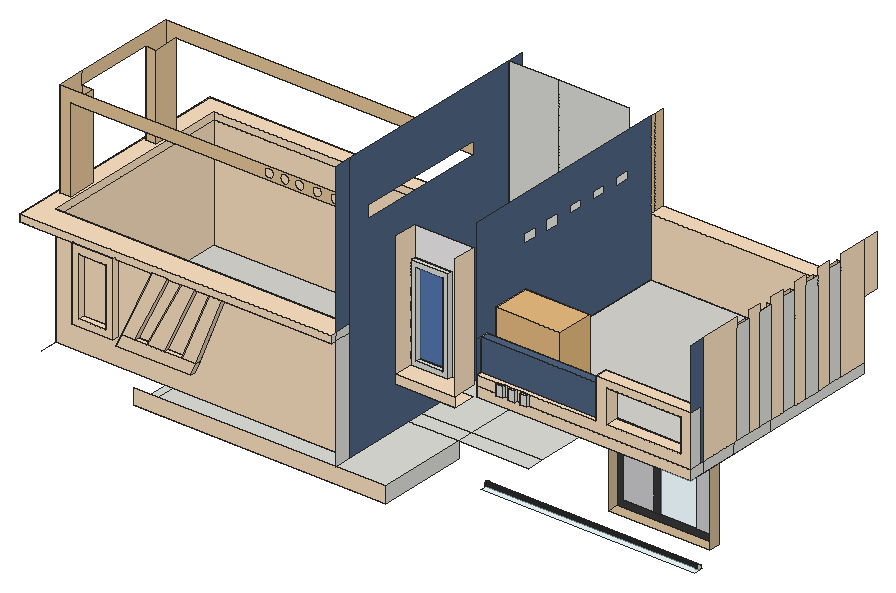
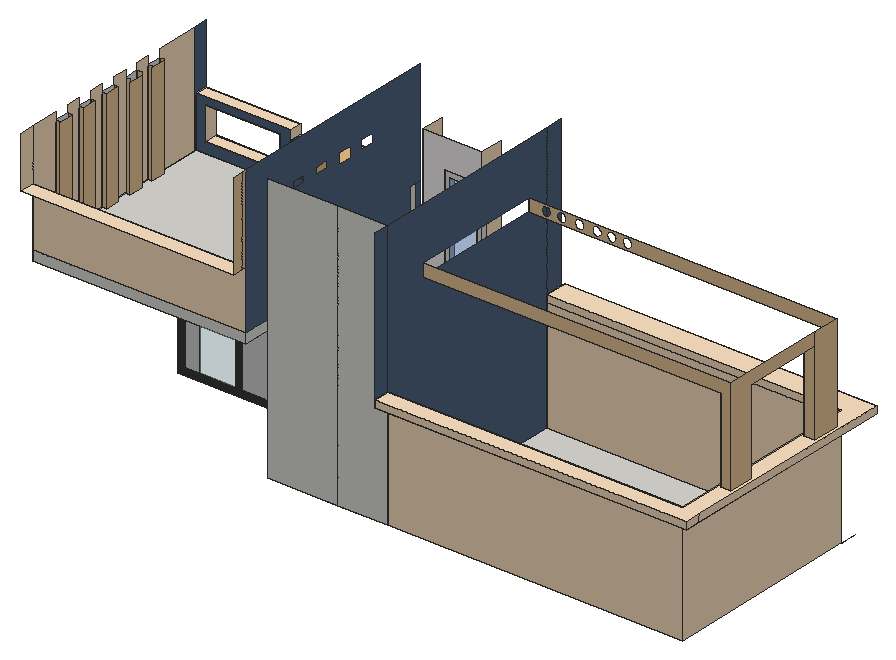
# SketchUp Ruby script. Lengths in inches.
U = 1.inch
M = Sketchup.active_model
def pt(a) = Geom::Point3d.new(a.map { |v| v * U })
def face(e, loops, mat)
  f = e.add_face(loops[0].map { |a| pt(a) })
  loops[1..].each { |l| e.add_face(l.map { |a| pt(a) }).erase! }
  f.material = f.back_material = mat if mat
  f
end
# faces: each face lists its corners as indices into pts; further lists are holes
def faces(e, pts, list, mat = nil) = list.each { |f| face(e, (f[0].is_a?(Array) ? f : [f]).map { |l| l.map { |i| pts[i] } }, mat) }
# xy, xz, yz: faces in a plane at the given z, y or x. An outline is a flat list of corners, or four numbers for a rectangle; further outlines are holes
def ring(l) = l.size == 4 ? [[l[0], l[1]], [l[2], l[1]], [l[2], l[3]], [l[0], l[3]]] : l.each_slice(2).to_a
def flat(e, list, mat, &to3) = list.each { |f| face(e, (f[0].is_a?(Array) ? f : [f]).map { |l| ring(l).map { |u, v| to3.(u, v) } }, mat) }
def xy(e, z, list, mat = nil) = flat(e, list, mat) { |x, y| [x, y, z] }
def xz(e, y, list, mat = nil) = flat(e, list, mat) { |x, z| [x, y, z] }
def yz(e, x, list, mat = nil) = flat(e, list, mat) { |y, z| [x, y, z] }
def lines(e, pts, list) = list.each { |a, b| e.add_line(pt(pts[a]), pt(pts[b])) }
# prism: a flat outline (further loops are holes) pulled along v
def prism(e, loops, v, mat = nil)
  f = face(e, loops, mat); d = Geom::Vector3d.new(v.map { |x| x * U })
  f.pushpull(f.normal.samedirection?(d) ? d.length : -d.length)
end
def box(e, o, s, mat = nil) = prism(e, [[o, [o[0] + s[0], o[1], o[2]], [o[0] + s[0], o[1] + s[1], o[2]], [o[0], o[1] + s[1], o[2]]]], [0, 0, s[2]], mat)
def at(x, y, z, deg = 0) = Geom::Transformation.translation(pt([x, y, z])) * Geom::Transformation.rotation(ORIGIN, Z_AXIS, deg.degrees)
def axes(o, x, y, z) = Geom::Transformation.new([*x, 0, *y, 0, *z, 0, *pt(o).to_a, 1])
def part(name) = M.definitions.add(name)
# library, detail: a bought-in or finely detailed component or shape, given as its bounding box
def library(name, o, s) = part(name).tap { |d| box(d.entities, o, s) }
def detail(e, o, s) = box(e.add_group.entities, o, s)
def put(e, d, t, mat = nil) = e.add_instance(d, t).tap { |i| i.material = mat if mat }
def group(e, t, mat = nil) = e.add_group.tap { |g| g.transformation = t; g.material = mat if mat }.entities
root = M.entities
M.materials.add("[0012_Bisque]").color = [255, 228, 196]
M.materials.add("[0035_Tan]").color = [234, 201, 156]
M.materials.add("[Blinds Vertical Pattern]1").color = [212, 212, 214]
M.materials.add("[Color M07]").color = [58, 58, 58]
M.materials.add("[Formica Beige]").color = [211, 187, 149]
M.materials.add("[Formica Graystone]").color = [149, 146, 135]
M.materials.add("[Leather Blue]").color = [80, 102, 132]
M.materials.add("[Stone Vein Gray]1").color = [247, 245, 245]
M.materials.add("[Terrazzo Tile Light]").color = [219, 217, 210]
M.materials.add("[Translucent Glass Blue]").color = [100, 149, 237]
M.materials["[Translucent Glass Blue]"].alpha = 0.5
M.materials.add("[Translucent Glass Safety]").color = [204, 235, 244]
M.materials["[Translucent Glass Safety]"].alpha = 0.5
c1 = library("Flora+17",[-57.52,158.6,-38.64],[66.99,62.88,77.28])
xy(root,862.4375,[[187.18,439.49,197.99,595.47],[197.99,439.49,607.9,595.47],[607.9,439.49,615.34,595.47],[138.99,595.47,228.43,623.86]])
xy(root,863.95,[[860.01,607.94,1033.1875,626.38]],"[Formica Beige]")
xy(root,889,[[529.97,439.49,615.34,595.47],[529.97,595.47,615.34,623.86],[615.34,595.47,733.59,623.86],[529.97,623.86,615.34,808.22],[615.34,623.86,733.59,808.22]])
xy(root,889,[[28.68,470.4375,529.97,808.22]],"[Terrazzo Tile Light]")
xy(root,933.85,[[771.27,448.03,1134.07,465.29]],"[Translucent Glass Safety]")
xy(root,947.54,[[162.87,431.49,290.72,439.49]],"[0012_Bisque]")
xy(root,956.62,[[89.49,428.49,159.99,439.49]],"[0012_Bisque]")
xy(root,967.96,[[172.3,431.49,195.38,439.49],[215.64,431.49,245.26,439.49],[274.875,431.49,298.76,439.49]])
xy(root,967.96,[[195.38,431.49,215.64,439.49],[245.26,431.49,274.875,439.49]],"[0012_Bisque]")
xy(root,968.65,[[101.71,428.49,147.77,439.49]],"[0012_Bisque]")
xy(root,1037.12,[[860.01,607.94,1033.1875,626.38]],"[Formica Beige]")
xy(root,1050.61,[[633.21,439.49,733.59,477.49]],"[0012_Bisque]")
xy(root,1067.2,[[633.21,470.42,696.47,478.61]])
xy(root,1067.2,[[633.21,439.49,733.59,439.49,733.59,478.61,696.47,478.61,696.47,470.42,633.21,470.42]],"[0012_Bisque]")
xy(root,1067.59,[[101.71,428.49,147.77,439.49]])
xy(root,1075.63,[[641.64,470.42,688.04,478.61]])
xy(root,1079.8125,[[89.49,428.49,159.99,431.49],[0,431.49,89.49,439.49],[89.49,431.49,159.99,439.49],[159.99,431.49,223.93,439.49],[223.93,431.49,250.55,439.49],
  [250.55,431.49,273.98,439.49],[273.98,431.49,297.72,439.49],[297.72,431.49,321.46,439.49],[321.46,431.49,342.79,439.49],[342.79,431.49,529.97,439.49],
  [0,439.49,0,835.03,529.97,835.03,529.97,808.22,28.68,808.22,28.68,470.4375,529.97,470.4375,529.97,439.49],[771.27,607.94,1134.07,808.22]])
xy(root,1079.8125,[[771.27,439.49,1134.07,607.94]],"[Leather Blue]")
xy(root,1092.125,[[[0,431.49,529.97,431.49,529.97,470.4375,28.68,470.4375,28.68,808.22,529.97,808.22,529.97,835.03,0,835.03],[5.5,509.25,23.8,555.46],[5.5,690.86,23.8,733.33]]],"[0012_Bisque]")
xy(root,1096.75,[[807.07,434.86,817.84,439.49],[827.75,434.86,838.53,439.49],[848.07,434.86,858.84,439.49],[771.27,439.49,1134.07,460.91],[1126.57,539.27,1134.07,560.75],
  [1126.57,560.75,1134.07,563.87],[1126.57,586.45,1134.07,607.94],[1126.57,607.94,1134.07,611.06],[1126.57,636.14,1134.07,660.75],[1126.57,685.02,1134.07,709.62],
  [1126.57,734.95,1134.07,759.56]])
xy(root,1096.75,[[771.27,460.91,1134.07,460.91,1134.07,539.27,1126.57,539.27,1126.57,563.87,1134.07,563.87,1134.07,586.45,1126.57,586.45,1126.57,611.06,1134.07,611.06,1134.07,636.14,1126.57,636.14,1126.57,660.75,1134.07,660.75,1134.07,685.02,1126.57,685.02,1126.57,709.62,1134.07,709.62,1134.07,734.95,1126.57,734.95,1126.57,759.56,1134.07,759.56,1134.07,808.22,771.27,808.22]],"[Terrazzo Tile Light]")
xy(root,1114.1875,[[807.07,434.86,817.84,439.49],[827.75,434.86,838.53,439.49],[848.07,434.86,858.84,439.49],[771.27,447.3,973.24,460.91]])
xy(root,1114.1875,[[771.27,439.49,973.24,447.3]],"[0012_Bisque]")
xy(root,1115.04,[[991.23,439.49,1117.66,460.91]],"[0012_Bisque]")
xy(root,1167.875,[[771.27,447.3,973.24,460.91]],"[Leather Blue]")
xy(root,1171.5,[[991.23,439.49,1117.66,460.91]])
xy(root,1182.875,[[973.24,439.49,1134.07,460.91]],"[0012_Bisque]")
xy(root,1197.6875,[[771.27,808.22,1134.07,835.03]],"[0012_Bisque]")
xy(root,1218.53,[[641.64,470.42,688.04,478.61]])
xy(root,1226.96,[[633.21,470.42,696.47,478.61]])
xz(root,428.49,[[[89.49,956.62,159.99,1079.8125],[101.71,968.65,147.77,1067.59]]],"[0012_Bisque]")
xz(root,431.49,[[162.87,947.54,290.72,947.54,298.76,967.96,172.3,967.96],[172.3,967.96,195.38,967.96,250.55,1079.8125,223.93,1079.8125],[215.64,967.96,245.26,967.96,297.72,1079.8125,273.98,1079.8125],[274.875,967.96,298.76,967.96,342.79,1079.8125,321.46,1079.8125],[0,1079.8125,529.97,1092.125]],"[0012_Bisque]")
xz(root,434.86,[[807.07,1096.75,817.84,1114.1875],[827.75,1096.75,838.53,1114.1875],[848.07,1096.75,858.84,1114.1875]])
xz(root,439.49,[[162.87,947.54,172.3,967.96,298.76,967.96,290.72,947.54],[[89.49,956.62,159.99,1079.8125],[101.71,968.65,147.77,1067.59]],[172.3,967.96,223.93,1079.8125,250.55,1079.8125,195.38,967.96],[215.64,967.96,273.98,1079.8125,297.72,1079.8125,245.26,967.96],[274.875,967.96,321.46,1079.8125,342.79,1079.8125,298.76,967.96],
  [807.07,1096.75,817.84,1114.1875],[827.75,1096.75,838.53,1114.1875],[848.07,1096.75,858.84,1114.1875]])
xz(root,439.49,[[187.18,862.4375,615.34,889],[195.38,967.96,215.64,967.96,273.98,1079.8125,250.55,1079.8125],[245.26,967.96,274.875,967.96,321.46,1079.8125,297.72,1079.8125],[101.71,968.65,147.77,1067.59],[633.21,1050.61,733.59,1067.2],
  [771.27,1079.8125,1134.07,1096.75],[771.27,1096.75,807.07,1114.1875],[817.84,1096.75,827.75,1114.1875],[838.53,1096.75,848.07,1114.1875],[[858.84,1096.75,1134.07,1096.75,1134.07,1182.875,973.24,1182.875,973.24,1114.1875,858.84,1114.1875],[991.23,1115.04,1117.66,1171.5]]],"[0012_Bisque]")
xz(root,447.3,[[771.27,1114.1875,973.24,1167.875]],"[Leather Blue]")
xz(root,460.91,[[[771.27,1096.75,771.27,1114.1875,973.24,1114.1875,973.24,1182.875,1134.07,1182.875,1134.07,1096.75],[991.23,1115.04,1117.66,1171.5]],[771.27,1114.1875,973.24,1167.875]],"[Leather Blue]")
xz(root,470.42,[[[633.21,1067.2,696.47,1226.96],[641.64,1075.63,688.04,1218.53]]])
xz(root,470.4375,[[28.68,889,529.97,1079.8125],[28.68,1079.8125,529.97,1092.125]],"[0012_Bisque]")
xz(root,478.61,[[[633.21,1067.2,696.47,1226.96],[641.64,1075.63,688.04,1218.53]]])
xz(root,478.61,[[696.47,1067.2,733.59,1067.2,733.59,1276.62,633.21,1276.62,633.21,1226.96,696.47,1226.96]],"[Stone Vein Gray]1")
xz(root,478.61,[[641.64,1075.63,688.04,1218.53]],"[Translucent Glass Blue]")
xz(root,509.25,[[[5.5,1092.125,23.8,1092.125,23.8,1235.23,529.97,1235.23,529.97,1256.625,5.5,1256.625],[473.26,1238.66,471.24,1238.93,469.35,1239.71,467.74,1240.95,466.49,1242.57,465.71,1244.45,465.45,1246.48,465.71,1248.5,466.49,1250.38,467.74,1252,469.35,1253.24,471.24,1254.02,473.26,1254.29,475.28,1254.02,477.17,1253.24,478.78,1252,480.03,1250.38,480.81,1248.5,481.07,1246.48,480.81,1244.45,480.03,1242.57,478.78,1240.95,477.17,1239.71,475.28,1238.93],[413.2,1238.66,411.18,1238.93,409.29,1239.71,407.67,1240.95,406.43,1242.57,405.65,1244.45,405.38,1246.48,405.65,1248.5,406.43,1250.38,407.67,1252,409.29,1253.24,411.18,1254.02,413.2,1254.29,415.22,1254.02,417.1,1253.24,418.72,1252,419.96,1250.38,420.74,1248.5,421.01,1246.48,420.74,1244.45,419.96,1242.57,418.72,1240.95,417.1,1239.71,415.22,1238.93],[442.88,1238.66,440.86,1238.93,438.98,1239.71,437.36,1240.95,436.12,1242.57,435.34,1244.45,435.07,1246.48,435.34,1248.5,436.12,1250.38,437.36,1252,438.98,1253.24,440.86,1254.02,442.88,1254.29,444.91,1254.02,446.79,1253.24,448.41,1252,449.65,1250.38,450.43,1248.5,450.7,1246.48,450.43,1244.45,449.65,1242.57,448.41,1240.95,446.79,1239.71,444.91,1238.93],[388.01,1238.66,385.99,1238.93,384.1,1239.71,382.49,1240.95,381.24,1242.57,380.46,1244.45,380.2,1246.48,380.46,1248.5,381.24,1250.38,382.49,1252,384.1,1253.24,385.99,1254.02,388.01,1254.29,390.03,1254.02,391.92,1253.24,393.53,1252,394.78,1250.38,395.56,1248.5,395.82,1246.48,395.56,1244.45,394.78,1242.57,393.53,1240.95,391.92,1239.71,390.03,1238.93],[499.45,1238.66,497.43,1238.93,495.54,1239.71,493.92,1240.95,492.68,1242.57,491.9,1244.45,491.63,1246.48,491.9,1248.5,492.68,1250.38,493.92,1252,495.54,1253.24,497.43,1254.02,499.45,1254.29,501.47,1254.02,503.35,1253.24,504.97,1252,506.21,1250.38,506.99,1248.5,507.26,1246.48,506.99,1244.45,506.21,1242.57,504.97,1240.95,503.35,1239.71,501.47,1238.93],[361.45,1238.66,359.43,1238.93,357.54,1239.71,355.92,1240.95,354.68,1242.57,353.9,1244.45,353.63,1246.48,353.9,1248.5,354.68,1250.38,355.92,1252,357.54,1253.24,359.43,1254.02,361.45,1254.29,363.47,1254.02,365.35,1253.24,366.97,1252,368.21,1250.38,368.99,1248.5,369.26,1246.48,368.99,1244.45,368.21,1242.57,366.97,1240.95,365.35,1239.71,363.47,1238.93]]],"[0035_Tan]")
xz(root,539.27,[[1126.57,1096.75,1134.07,1271.79]],"[0035_Tan]")
xz(root,555.46,[[5.5,1092.125,23.8,1235.23]],"[0035_Tan]")
xz(root,563.87,[[1126.57,1096.75,1134.07,1271.79]],"[0035_Tan]")
xz(root,586.45,[[1126.57,1096.75,1134.07,1272.79]],"[0035_Tan]")
xz(root,611.06,[[1126.57,1096.75,1134.07,1272.79]],"[0035_Tan]")
xz(root,626.38,[[871.74,875.67,922.51,1025.4],[996.07,875.67,1021.47,1025.4]],"[Blinds Vertical Pattern]1")
xz(root,626.38,[[[860.01,863.95,1033.1875,1037.12],[871.74,875.67,1021.47,1025.4]],[922.51,875.67,933.66,1025.4]],"[Color M07]")
xz(root,626.38,[[933.66,875.67,996.07,1025.4]],"[Translucent Glass Safety]")
xz(root,636.14,[[1126.57,1096.75,1134.07,1272.79]],"[0035_Tan]")
xz(root,660.75,[[1126.57,1096.75,1134.07,1272.79]],"[0035_Tan]")
xz(root,685.02,[[1126.57,1096.75,1134.07,1272.79]],"[0035_Tan]")
xz(root,690.86,[[5.5,1092.125,23.8,1235.23]],"[0035_Tan]")
xz(root,709.62,[[1126.57,1096.75,1134.07,1272.79]],"[0035_Tan]")
xz(root,733.33,[[5.5,1092.125,5.5,1256.625,529.97,1256.625,529.97,1235.23,23.8,1235.23,23.8,1092.125]],"[0035_Tan]")
xz(root,734.95,[[1126.57,1096.75,1134.07,1272.79]],"[0035_Tan]")
xz(root,759.56,[[1126.57,1096.75,1134.07,1272.79]],"[0035_Tan]")
xz(root,808.22,[[529.97,889,615.34,1345.9375],[615.34,889,733.59,1345.9375],[771.27,1079.8125,1134.07,1096.75]])
xz(root,808.22,[[28.68,889,529.97,1079.8125],[28.68,1079.8125,529.97,1092.125],[771.27,1096.75,1134.07,1197.6875]],"[0012_Bisque]")
xz(root,835.03,[[0,1079.8125,529.97,1092.125]],"[0012_Bisque]")
yz(root,0,[[431.49,1079.8125,808.22,1092.125],[808.22,1079.8125,835.03,1092.125]],"[0012_Bisque]")
yz(root,5.5,[[509.25,1092.125,555.46,1256.625],[690.86,1092.125,690.86,1235.23,555.46,1235.23,555.46,1256.625,733.33,1256.625,733.33,1092.125]],"[0035_Tan]")
yz(root,23.8,[[509.25,1092.125,555.46,1235.23],[690.86,1092.125,733.33,1235.23]],"[0035_Tan]")
yz(root,28.68,[[470.4375,889,808.22,1079.8125],[470.4375,1079.8125,808.22,1092.125]],"[0012_Bisque]")
yz(root,89.49,[[428.49,956.62,439.49,1079.8125]],"[0012_Bisque]")
yz(root,101.71,[[428.49,968.65,439.49,1067.59]],"[0012_Bisque]")
yz(root,147.77,[[428.49,968.65,439.49,1067.59]],"[0012_Bisque]")
yz(root,159.99,[[428.49,956.62,439.49,1079.8125]],"[0012_Bisque]")
yz(root,529.97,[[439.49,889,470.4375,1079.8125],[431.49,1079.8125,439.49,1092.125],[439.49,1079.8125,470.4375,1092.125],[808.22,1079.8125,835.03,1092.125]])
yz(root,529.97,[[[470.4375,889,808.22,1345.9375],[509.25,1235.23,733.33,1256.625]],[439.49,1092.125,470.4375,1345.9375],[808.22,1092.125,835.03,1345.9375]],"[Leather Blue]")
yz(root,615.34,[[439.49,862.4375,595.47,889]])
yz(root,633.21,[[470.42,1067.2,478.61,1226.96]])
yz(root,633.21,[[439.49,1067.2,470.42,1067.2,470.42,1226.96,478.61,1226.96,478.61,1276.62,439.49,1276.62]],"[0012_Bisque]")
yz(root,641.64,[[470.42,1075.63,478.61,1218.53]])
yz(root,688.04,[[470.42,1075.63,478.61,1218.53]])
yz(root,696.47,[[470.42,1067.2,478.61,1226.96]])
yz(root,733.59,[[439.49,1067.2,478.61,1276.62]],"[0012_Bisque]")
yz(root,771.27,[[439.49,1079.8125,808.22,1096.75],[439.49,1096.75,460.91,1114.1875],[447.3,1114.1875,460.91,1167.875]])
yz(root,771.27,[[808.22,1197.6875,817.66,1345.9375],[817.66,1197.6875,835.03,1345.9375]],"[0035_Tan]")
yz(root,771.27,[[[460.91,1096.75,808.22,1096.75,808.22,1345.9375,439.49,1345.9375,439.49,1167.875,460.91,1167.875],[586.45,1266.48,611.06,1284.8125],[539.27,1268.97,563.87,1284.8125],[734.95,1271.04,759.56,1284.8125],[636.14,1272.79,660.75,1284.8125],[685.02,1272.79,709.62,1284.8125]],[439.49,1114.1875,447.3,1167.875]],"[Leather Blue]")
yz(root,807.07,[[434.86,1096.75,439.49,1114.1875]])
yz(root,817.84,[[434.86,1096.75,439.49,1114.1875]])
yz(root,827.75,[[434.86,1096.75,439.49,1114.1875]])
yz(root,838.53,[[434.86,1096.75,439.49,1114.1875]])
yz(root,848.07,[[434.86,1096.75,439.49,1114.1875]])
yz(root,858.84,[[434.86,1096.75,439.49,1114.1875]])
yz(root,860.01,[[607.94,863.95,626.38,1037.12]],"[Formica Beige]")
yz(root,973.24,[[447.3,1114.1875,460.91,1167.875]])
yz(root,973.24,[[439.49,1114.1875,447.3,1167.875],[439.49,1167.875,460.91,1182.875]],"[0012_Bisque]")
yz(root,991.23,[[439.49,1115.04,460.91,1171.5]],"[0012_Bisque]")
yz(root,1033.1875,[[607.94,863.95,626.38,1037.12]],"[Formica Beige]")
yz(root,1117.66,[[439.49,1115.04,460.91,1171.5]],"[0012_Bisque]")
yz(root,1126.57,[[539.27,1096.75,563.87,1268.97],[586.45,1096.75,611.06,1266.48],[636.14,1096.75,660.75,1272.79],[685.02,1096.75,709.62,1272.79],[734.95,1096.75,759.56,1271.04]],"[0035_Tan]")
yz(root,1134.07,[[458.49,936.6,459.3,936.71,460.05,937.02,460.7,937.51,461.19,938.16,461.51,938.92,461.61,939.72,461.51,940.53,461.19,941.29,460.7,941.93,460.05,942.43,459.3,942.74,458.49,942.85,457.68,942.74,456.93,942.43,456.28,941.93,455.78,941.29,455.47,940.53,455.36,939.72,455.47,938.92,455.78,938.16,456.28,937.51,456.93,937.02,457.68,936.71],[439.49,1079.8125,466.29,1096.75],[466.29,1079.8125,532.66,1096.75],[532.66,1079.8125,607.94,1096.75],[607.94,1079.8125,808.22,1096.75],
  [439.49,1096.75,460.91,1182.875],[539.27,1096.75,563.87,1271.79],[586.45,1096.75,611.06,1272.79],[636.14,1096.75,660.75,1272.79],[685.02,1096.75,709.62,1272.79],
  [734.95,1096.75,759.56,1272.79]])
yz(root,1134.07,[[466.29,1096.75,539.27,1284.8125],[563.87,1096.75,586.45,1284.8125],[611.06,1096.75,636.14,1284.8125],[660.75,1096.75,685.02,1284.8125],[709.62,1096.75,734.95,1284.8125],
  [759.56,1096.75,808.22,1284.8125],[808.22,1197.6875,835.03,1284.8125]],"[0012_Bisque]")
yz(root,1134.07,[[460.91,1096.75,460.91,1182.875,439.49,1182.875,439.49,1284.8125,466.29,1284.8125,466.29,1096.75]],"[Leather Blue]")
p = [[1134.07,458.49,936.6],[1134.07,457.68,936.71],[771.27,457.68,936.71],[771.27,458.49,936.6],[1134.07,459.3,936.71],[771.27,459.3,936.71],
  [1134.07,456.93,937.02],[771.27,456.93,937.02],[1134.07,460.05,937.02],[771.27,460.05,937.02],[1134.07,456.28,937.51],[771.27,456.28,937.51],
  [1134.07,460.7,937.51],[771.27,460.7,937.51],[1134.07,455.78,938.16],[771.27,455.78,938.16],[1134.07,461.19,938.16],[771.27,461.19,938.16],
  [1134.07,455.47,938.92],[771.27,455.47,938.92],[1134.07,461.51,938.92],[771.27,461.51,938.92],[1134.07,455.36,939.72],[771.27,455.36,939.72],
  [1134.07,461.61,939.72],[771.27,461.61,939.72],[1134.07,455.47,940.53],[771.27,455.47,940.53],[1134.07,461.51,940.53],[771.27,461.51,940.53],
  [1134.07,455.78,941.29],[771.27,455.78,941.29],[1134.07,461.19,941.29],[771.27,461.19,941.29],[1134.07,456.28,941.93],[771.27,456.28,941.93],
  [1134.07,460.7,941.93],[771.27,460.7,941.93],[1134.07,456.93,942.43],[771.27,456.93,942.43],[1134.07,460.05,942.43],[771.27,460.05,942.43],
  [1134.07,457.68,942.74],[771.27,457.68,942.74],[1134.07,459.3,942.74],[771.27,459.3,942.74],[1134.07,458.49,942.85],[771.27,458.49,942.85],
  [172.3,439.49,967.96],[162.87,439.49,947.54],[162.87,431.49,947.54],[172.3,431.49,967.96],[290.72,439.49,947.54],[298.76,439.49,967.96],
  [298.76,431.49,967.96],[290.72,431.49,947.54],[223.93,439.49,1079.8125],[223.93,431.49,1079.8125],[195.38,439.49,967.96],[250.55,439.49,1079.8125],
  [250.55,431.49,1079.8125],[195.38,431.49,967.96],[273.98,439.49,1079.8125],[215.64,439.49,967.96],[215.64,431.49,967.96],[273.98,431.49,1079.8125],
  [245.26,439.49,967.96],[297.72,439.49,1079.8125],[297.72,431.49,1079.8125],[245.26,431.49,967.96],[321.46,439.49,1079.8125],[274.875,439.49,967.96],
  [274.875,431.49,967.96],[321.46,431.49,1079.8125],[342.79,439.49,1079.8125],[342.79,431.49,1079.8125],[228.43,623.86,862.4375],[228.43,623.86,889],
  [28.68,470.4375,889],[28.68,439.49,889]]
faces(root,p,[[0,1,2,3],[4,0,3,5],[1,6,7,2],[8,4,5,9],[6,10,11,7],[12,8,9,13],[10,14,15,11],[16,12,13,17],
  [14,18,19,15],[20,16,17,21],[18,22,23,19],[24,20,21,25],[22,26,27,23],[28,24,25,29],[26,30,31,27],[32,28,29,33],
  [30,34,35,31],[36,32,33,37],[34,38,39,35],[40,36,37,41],[38,42,43,39],[44,40,41,45],[42,46,47,43],[46,44,45,47]],"[Formica Graystone]")
faces(root,p,[[48,49,50,51],[52,53,54,55],[56,48,51,57],[58,59,60,61],[62,63,64,65],[66,67,68,69],[70,71,72,73],[53,74,75,54]],"[0012_Bisque]")
lines(root,p,[[76,77],[78,79]])
put(root,c1,axes([874.26,309.375,1151.93],[1.638,0,0],[0,1,0],[0,0,1.428]))
